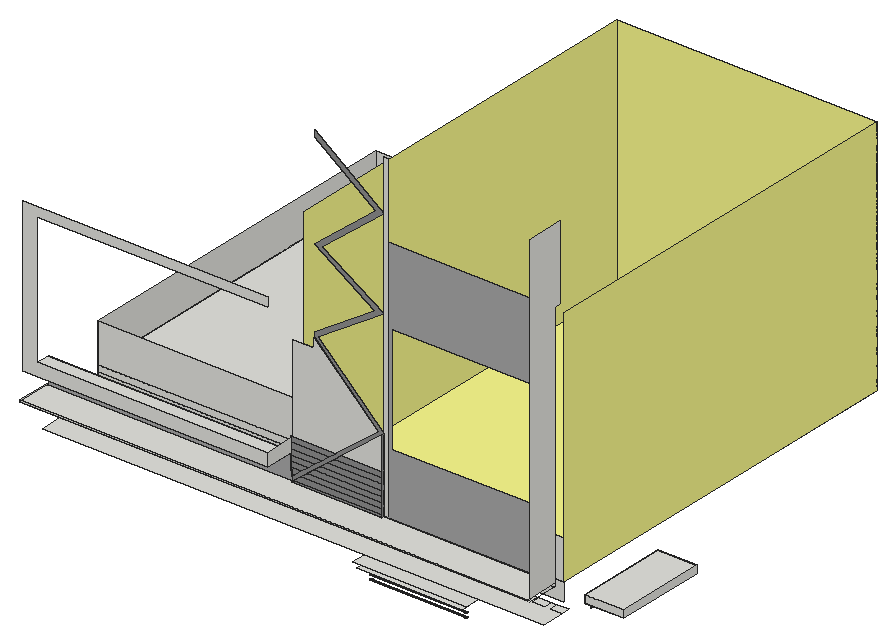
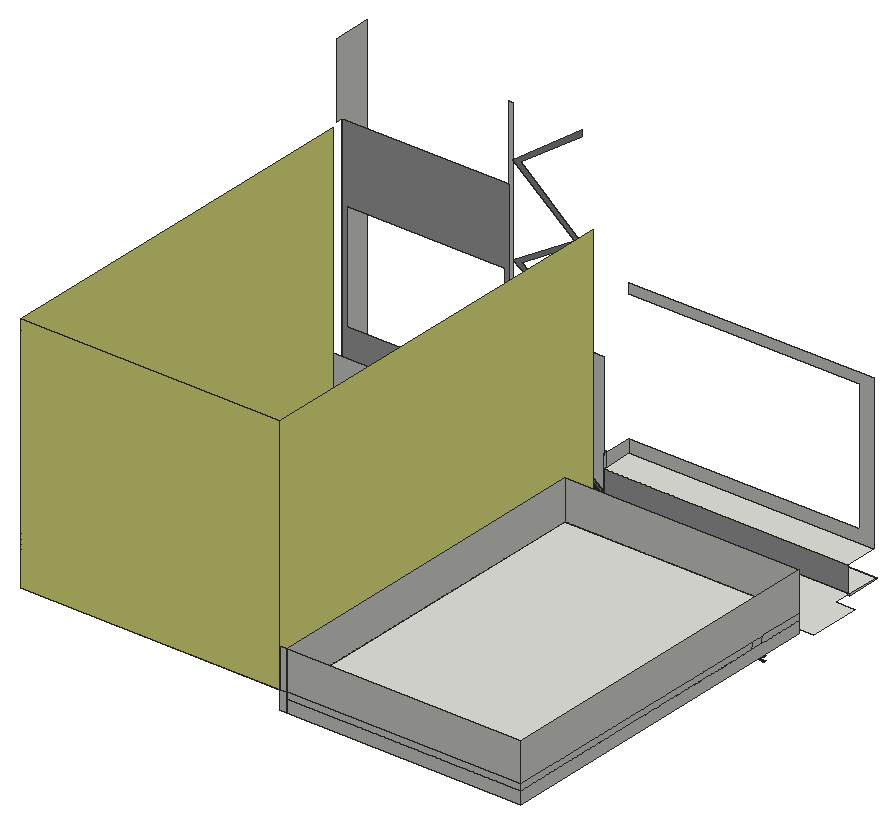
# SketchUp Ruby script. Lengths in inches.
U = 1.inch
M = Sketchup.active_model
def pt(a) = Geom::Point3d.new(a.map { |v| v * U })
def face(e, loops, mat)
  f = e.add_face(loops[0].map { |a| pt(a) })
  loops[1..].each { |l| e.add_face(l.map { |a| pt(a) }).erase! }
  f.material = f.back_material = mat if mat
  f
end
# faces: each face lists its corners as indices into pts; further lists are holes
def faces(e, pts, list, mat = nil) = list.each { |f| face(e, (f[0].is_a?(Array) ? f : [f]).map { |l| l.map { |i| pts[i] } }, mat) }
# xy, xz, yz: faces in a plane at the given z, y or x. An outline is a flat list of corners, or four numbers for a rectangle; further outlines are holes
def ring(l) = l.size == 4 ? [[l[0], l[1]], [l[2], l[1]], [l[2], l[3]], [l[0], l[3]]] : l.each_slice(2).to_a
def flat(e, list, mat, &to3) = list.each { |f| face(e, (f[0].is_a?(Array) ? f : [f]).map { |l| ring(l).map { |u, v| to3.(u, v) } }, mat) }
def xy(e, z, list, mat = nil) = flat(e, list, mat) { |x, y| [x, y, z] }
def xz(e, y, list, mat = nil) = flat(e, list, mat) { |x, z| [x, y, z] }
def yz(e, x, list, mat = nil) = flat(e, list, mat) { |y, z| [x, y, z] }
def lines(e, pts, list) = list.each { |a, b| e.add_line(pt(pts[a]), pt(pts[b])) }
# prism: a flat outline (further loops are holes) pulled along v
def prism(e, loops, v, mat = nil)
  f = face(e, loops, mat); d = Geom::Vector3d.new(v.map { |x| x * U })
  f.pushpull(f.normal.samedirection?(d) ? d.length : -d.length)
end
def box(e, o, s, mat = nil) = prism(e, [[o, [o[0] + s[0], o[1], o[2]], [o[0] + s[0], o[1] + s[1], o[2]], [o[0], o[1] + s[1], o[2]]]], [0, 0, s[2]], mat)
def at(x, y, z, deg = 0) = Geom::Transformation.translation(pt([x, y, z])) * Geom::Transformation.rotation(ORIGIN, Z_AXIS, deg.degrees)
def axes(o, x, y, z) = Geom::Transformation.new([*x, 0, *y, 0, *z, 0, *pt(o).to_a, 1])
def part(name) = M.definitions.add(name)
# library, detail: a bought-in or finely detailed component or shape, given as its bounding box
def library(name, o, s) = part(name).tap { |d| box(d.entities, o, s) }
def detail(e, o, s) = box(e.add_group.entities, o, s)
def put(e, d, t, mat = nil) = e.add_instance(d, t).tap { |i| i.material = mat if mat }
def group(e, t, mat = nil) = e.add_group.tap { |g| g.transformation = t; g.material = mat if mat }.entities
root = M.entities
M.materials.add("[0032_Moccasin]").color = [249, 249, 141]
M.materials.add("[0132_LightGray]").color = [169, 169, 169]
M.materials.add("[Color M04]").color = [142, 142, 142]
M.materials.add("[Wood Bamboo]").color = [195, 96, 5]
M.materials.add("[Wood Cherry Original]").color = [152, 68, 0]
M.materials.add("[Wood Cherry Original]1").color = [152, 86, 42]
xy(root,126,[[149.49,84.25,191.49,85.25]],"[Wood Cherry Original]")
xy(root,136.59,[[316.01,39.5625,334.01,43],[334.01,39.5625,340.01,40.5625],[340.01,39.5625,381.26,43],[381.26,39.5625,387.26,40.5625],[387.26,39.5625,405.26,43]],"[Wood Bamboo]")
xy(root,137.01,[[103.25,82.25,107.25,84.25]])
xy(root,137.01,[[61.9375,82.25,103.25,84.25],[107.25,82.25,119.25,84.25]],"[Wood Cherry Original]")
xy(root,140.59,[[312.01,30.4375,409.26,39.5625],[312.01,39.5625,409.26,43],[312.01,43,409.26,50.6875]])
xy(root,141.01,[[57.9375,82.25,123.25,84.25]],"[Wood Cherry Original]1")
xy(root,144.4,[[308.2,30.4375,413.0625,44.6875]])
xy(root,155,[[495.875,70.375,496.875,140.375]])
xy(root,162,[[495.875,63.375,496.875,147.375],[[496.875,63.375,531.875,147.375],[513.08,87.9375,514.63,88.14,516.08,88.74,517.32,89.7,518.28,90.9375,518.875,92.39,519.08,93.9375,518.875,95.49,518.28,96.9375,517.32,98.18,516.08,99.14,514.63,99.73,513.08,99.9375,511.53,99.73,510.08,99.14,508.84,98.18,507.88,96.9375,507.29,95.49,507.08,93.9375,507.29,92.39,507.88,90.9375,508.84,89.7,510.08,88.74,511.53,88.14]],[513.08,87.9375,511.53,88.14,510.08,88.74,508.84,89.7,507.88,90.9375,507.29,92.39,507.08,93.9375,507.29,95.49,507.88,96.9375,508.84,98.18,510.08,99.14,511.53,99.73,513.08,99.9375,514.63,99.73,516.08,99.14,517.32,98.18,518.28,96.9375,518.875,95.49,519.08,93.9375,518.875,92.39,518.28,90.9375,517.32,89.7,516.08,88.74,514.63,88.14]])
xy(root,165,[[33.875,15.6875,33.875,36.73,15.875,36.73,15.875,84.25,213.63,84.25,213.63,36.625,225.4375,36.625,225.4375,49.4375,230.75,49.4375,230.75,36.625,241.25,36.625,241.25,44.6875,468.26,44.6875,468.26,36.625,480.0625,36.625,480.0625,44.6875,485.375,44.6875,485.375,36.625,495.875,36.625,495.875,15.6875],[213.63,36.625,225.4375,84.25],[230.75,36.625,241.25,84.25],[468.26,36.625,480.0625,44.6875],[485.375,36.625,495.875,44.6875],
  [225.4375,49.4375,230.75,84.25]])
xy(root,169,[[495.875,63.375,531.875,147.375]])
xy(root,176,[[24.875,90.25,241.25,411]])
xy(root,180.75,[[14.3125,14.25,14.3125,44.6875,15.875,44.6875,15.875,15.6875,482.9375,15.6875,482.9375,14.25]])
xy(root,182,[[14.3125,14.25,482.9375,14.25,482.9375,44.6875,325.49,44.6875,325.49,42.75,241.89,42.75,241.89,44.6875,14.3125,44.6875],[241.89,42.75,325.49,44.6875],[241.89,44.6875,325.49,46.6875],[241.89,46.6875,241.89,52.125,247.25,52.125,247.25,50.6875,325.49,50.6875,325.49,46.6875],[247.25,50.6875,325.49,52.125],
  [24.875,90.25,241.25,411]])
xy(root,182,[[325.49,50.6875,486.875,50.6875,486.875,411,247.25,411,247.25,52.125,325.49,52.125]],"[0032_Moccasin]")
xy(root,205.89,[[15.875,15.6875,241.25,44.6875]])
xz(root,14.25,[[14.3125,180.75,482.9375,182]])
xz(root,15.6875,[[15.875,205.89,241.25,205.89,241.25,218,28.03,218,28.03,338,241.25,338,241.25,347,15.875,347]])
xz(root,42.75,[[241.89,182,325.49,182,325.49,183.79,244.08,183.79],[244.08,183.79,325.49,183.79,325.49,188.92,250.33,188.92],[241.76,186.7,244.49,188.92,241.7,188.92],[241.7,188.92,244.49,188.92,250.79,194.04,241.57,194.04],[250.33,188.92,325.49,188.92,325.49,194.04,256.59,194.04],
  [241.57,194.04,250.79,194.04,257.1,199.17,241.43,199.17],[256.59,194.04,325.49,194.04,325.49,199.17,262.85,199.17],[241.43,199.17,257.1,199.17,263.4,204.29,241.29,204.29],[262.85,199.17,325.49,199.17,325.49,204.29,269.11,204.29],[241.29,204.29,263.4,204.29,269.7,209.42,241.25,209.42,241.25,205.89],
  [269.11,204.29,325.49,204.29,325.49,209.42,275.37,209.42],[241.25,209.42,269.7,209.42,276,214.54,241.25,214.54],[275.37,209.42,325.49,209.42,325.49,214.54,281.625,214.54],[241.25,214.54,276,214.54,282.3,219.67,241.25,219.67],[281.625,214.54,325.49,214.54,325.49,219.67,287.88,219.67]],"[Color M04]")
xz(root,44.4375,[[241.76,186.7,241.25,205.89,241.25,298.5,261.37,298.5,261.37,306.96,319.9,250.25]])
xz(root,44.6875,[[325.49,179.25,329.48,182],[329.48,179.25,482.9375,182],[14.3125,180.75,15.875,182],[241.89,182,325.49,250.46,325.49,182],[325.49,182,329.48,479],
  [241.76,186.7,241.25,205.89,241.25,298.5,261.37,298.5,261.37,306.96,319.9,250.25]])
xz(root,44.6875,[[15.875,182,241.89,182,241.76,186.7,241.25,205.89,15.875,205.89],[[329.48,182,482.9375,410],[333.13,239.94,333.13,337.75,332.44,337.75,332.44,339.8125,478.87,339.8125,478.87,337.75,478.31,337.75,478.31,239.94]]],"[0132_LightGray]")
xz(root,44.6875,[[241.89,182,325.49,250.46,264.35,308.92,325.49,349.15,268.3,384.6,325.49,431.84,261.37,479,261.37,473.32,318.21,432.15,261.37,384.6,317.38,349.1,261.37,311.77,261.37,306.96,319.9,250.25,241.76,186.7]],"[Color M04]")
xz(root,46.6875,[[241.89,182,325.49,250.46,325.49,182]])
xz(root,50.6875,[[247.25,165,377.96,182],[377.96,165,403.71,182],[403.71,165,486.875,182],[247.25,182,486.875,218]])
xz(root,52.125,[[241.89,182,325.49,250.46,325.49,182]])
xz(root,63.375,[[495.875,162,531.875,169]])
xz(root,90.25,[[24.875,165,241.25,176],[24.875,176,241.25,182],[24.875,182,241.25,218]])
xz(root,147.375,[[495.875,162,531.875,169]])
xz(root,411,[[24.875,165,241.25,176],[241.25,165,247.25,182],[24.875,176,241.25,182],[24.875,182,241.25,218],[241.25,182,247.25,218]])
xz(root,411,[[247.25,182,486.875,404]],"[0032_Moccasin]")
yz(root,14.3125,[[14.25,180.75,44.6875,182]])
yz(root,24.875,[[90.25,165,411,176],[90.25,176,132.85,182],[132.85,176,144.6,182],[144.6,176,411,182],[90.25,182,411,218]])
yz(root,241.25,[[90.25,165,411,176],[90.25,176,411,182],[90.25,182,411,218],[15.6875,205.89,42.75,218],[42.75,205.89,44.4375,218],
  [44.4375,205.89,44.6875,218]])
yz(root,247.25,[[50.6875,182,411,404]],"[0032_Moccasin]")
yz(root,325.49,[[44.6875,182,46.6875,250.46],[46.6875,182,52.125,250.46]])
yz(root,325.49,[[42.75,182,44.6875,250.46]],"[Color M04]")
yz(root,482.9375,[[14.25,180.75,15.6875,182],[15.6875,182,15.6875,479,50.6875,479,50.6875,410,44.6875,410,44.6875,182]])
yz(root,486.875,[[50.6875,182,411,404]],"[0032_Moccasin]")
yz(root,495.875,[[63.375,162,147.375,169]])
yz(root,531.875,[[63.375,162,147.375,169]])
p = [[119.25,83,126.03],[119.25,82.9,126.11],[61.9375,82.9,126.11],[61.9375,83,126.03],[119.25,83.12,125.98],[61.9375,83.12,125.98],
  [119.25,83.25,125.96],[61.9375,83.25,125.96],[119.25,83.38,125.98],[61.9375,83.38,125.98],[119.25,83.5,126.03],[61.9375,83.5,126.03],
  [119.25,83.6,126.11],[61.9375,83.6,126.11],[119.25,82.82,126.21],[61.9375,82.82,126.21],[119.25,83.68,126.21],[61.9375,83.68,126.21],
  [119.25,82.77,126.34],[61.9375,82.77,126.34],[119.25,83.73,126.34],[61.9375,83.73,126.34],[119.25,82.75,126.46],[61.9375,82.75,126.46],
  [119.25,83.75,126.46],[61.9375,83.75,126.46],[119.25,82.77,126.59],[61.9375,82.77,126.59],[119.25,83.73,126.59],[61.9375,83.73,126.59],
  [119.25,82.82,126.71],[61.9375,82.82,126.71],[119.25,83.68,126.71],[61.9375,83.68,126.71],[119.25,82.9,126.82],[61.9375,82.9,126.82],
  [119.25,83.6,126.82],[61.9375,83.6,126.82],[119.25,83,126.9],[61.9375,83,126.9],[119.25,83.5,126.9],[61.9375,83.5,126.9],
  [119.25,83.12,126.95],[61.9375,83.12,126.95],[119.25,83.25,126.96],[61.9375,83.25,126.96],[119.25,83.38,126.95],[61.9375,83.38,126.95],
  [316.01,41.03,127.78],[316.01,41.15,127.73],[405.26,41.15,127.73],[405.26,41.03,127.78],[316.01,41.28,127.71],[405.26,41.28,127.71],
  [316.01,41.41,127.73],[405.26,41.41,127.73],[316.01,41.53,127.78],[405.26,41.53,127.78],[316.01,40.93,127.86],[405.26,40.93,127.86],
  [316.01,41.63,127.86],[405.26,41.63,127.86],[316.01,40.85,127.96],[405.26,40.85,127.96],[316.01,41.71,127.96],[405.26,41.71,127.96],
  [316.01,40.8,128.08],[405.26,40.8,128.08],[316.01,41.76,128.08],[405.26,41.76,128.08],[316.01,40.78,128.21],[405.26,40.78,128.21],
  [316.01,41.78,128.21],[405.26,41.78,128.21],[316.01,40.8,128.34],[405.26,40.8,128.34],[316.01,41.76,128.34],[405.26,41.76,128.34],
  [316.01,40.85,128.46],[405.26,40.85,128.46],[316.01,41.71,128.46],[405.26,41.71,128.46],[316.01,40.93,128.57],[405.26,40.93,128.57],
  [316.01,41.63,128.57],[405.26,41.63,128.57],[316.01,41.03,128.65],[405.26,41.03,128.65],[316.01,41.15,128.7],[405.26,41.15,128.7],
  [316.01,41.53,128.65],[316.01,41.41,128.7],[405.26,41.41,128.7],[405.26,41.53,128.65],[316.01,41.28,128.71],[405.26,41.28,128.71],
  [119.25,83,130.03],[119.25,82.9,130.11],[61.9375,82.9,130.11],[61.9375,83,130.03],[119.25,83.12,129.98],[61.9375,83.12,129.98],
  [119.25,83.25,129.96],[61.9375,83.25,129.96],[119.25,83.38,129.98],[61.9375,83.38,129.98],[119.25,83.5,130.03],[61.9375,83.5,130.03],
  [119.25,83.6,130.11],[61.9375,83.6,130.11],[119.25,82.82,130.21],[61.9375,82.82,130.21],[119.25,83.68,130.21],[61.9375,83.68,130.21],
  [119.25,82.77,130.34],[61.9375,82.77,130.34],[119.25,83.73,130.34],[61.9375,83.73,130.34],[119.25,82.75,130.46],[61.9375,82.75,130.46],
  [119.25,83.75,130.46],[61.9375,83.75,130.46],[119.25,82.77,130.59],[61.9375,82.77,130.59],[119.25,83.73,130.59],[61.9375,83.73,130.59],
  [119.25,82.82,130.71],[61.9375,82.82,130.71],[119.25,83.68,130.71],[61.9375,83.68,130.71],[119.25,82.9,130.82],[61.9375,82.9,130.82],
  [119.25,83.6,130.82],[61.9375,83.6,130.82],[119.25,83,130.9],[61.9375,83,130.9],[119.25,83.5,130.9],[61.9375,83.5,130.9],
  [119.25,83.12,130.95],[61.9375,83.12,130.95],[119.25,83.25,130.96],[61.9375,83.25,130.96],[119.25,83.38,130.95],[61.9375,83.38,130.95],
  [316.01,41.03,131.78],[316.01,41.15,131.73],[405.26,41.15,131.73],[405.26,41.03,131.78],[316.01,41.28,131.71],[405.26,41.28,131.71],
  [316.01,41.41,131.73],[405.26,41.41,131.73],[316.01,41.53,131.78],[405.26,41.53,131.78],[316.01,40.93,131.86],[405.26,40.93,131.86],
  [316.01,41.63,131.86],[405.26,41.63,131.86],[316.01,40.85,131.96],[405.26,40.85,131.96],[316.01,41.71,131.96],[405.26,41.71,131.96],
  [316.01,40.8,132.08],[405.26,40.8,132.08],[316.01,41.76,132.08],[405.26,41.76,132.08],[316.01,40.78,132.21],[405.26,40.78,132.21],
  [316.01,41.78,132.21],[405.26,41.78,132.21],[316.01,40.8,132.34],[405.26,40.8,132.34],[316.01,41.76,132.34],[405.26,41.76,132.34],
  [316.01,40.85,132.46],[405.26,40.85,132.46],[316.01,41.71,132.46],[405.26,41.71,132.46],[316.01,40.93,132.57],[405.26,40.93,132.57],
  [316.01,41.63,132.57],[405.26,41.63,132.57],[316.01,41.03,132.65],[405.26,41.03,132.65],[316.01,41.15,132.7],[405.26,41.15,132.7],
  [316.01,41.53,132.65],[316.01,41.41,132.7],[405.26,41.41,132.7],[405.26,41.53,132.65],[316.01,41.28,132.71],[405.26,41.28,132.71],
  [119.25,83,134.03],[119.25,82.9,134.11],[61.9375,82.9,134.11],[61.9375,83,134.03],[119.25,83.12,133.98],[61.9375,83.12,133.98],
  [119.25,83.25,133.96],[61.9375,83.25,133.96],[119.25,83.38,133.98],[61.9375,83.38,133.98],[119.25,83.5,134.03],[61.9375,83.5,134.03],
  [119.25,83.6,134.11],[61.9375,83.6,134.11],[119.25,82.82,134.21],[61.9375,82.82,134.21],[119.25,83.68,134.21],[61.9375,83.68,134.21],
  [119.25,82.77,134.34],[61.9375,82.77,134.34],[119.25,83.73,134.34],[61.9375,83.73,134.34],[119.25,82.75,134.46],[61.9375,82.75,134.46],
  [119.25,83.75,134.46],[61.9375,83.75,134.46],[119.25,82.77,134.59],[61.9375,82.77,134.59],[119.25,83.73,134.59],[61.9375,83.73,134.59],
  [119.25,82.82,134.71],[61.9375,82.82,134.71],[119.25,83.68,134.71],[61.9375,83.68,134.71],[119.25,82.9,134.82],[61.9375,82.9,134.82],
  [119.25,83.6,134.82],[61.9375,83.6,134.82],[119.25,83,134.9],[61.9375,83,134.9],[119.25,83.5,134.9],[61.9375,83.5,134.9],
  [119.25,83.12,134.95],[61.9375,83.12,134.95],[119.25,83.25,134.96],[61.9375,83.25,134.96],[119.25,83.38,134.95],[61.9375,83.38,134.95],
  [325.49,44.6875,250.46],[241.89,44.6875,182],[241.89,42.75,182],[244.08,42.75,183.79],[250.33,42.75,188.92],[256.59,42.75,194.04],
  [262.85,42.75,199.17],[269.11,42.75,204.29],[275.37,42.75,209.42],[281.625,42.75,214.54],[287.88,42.75,219.67],[294.14,42.75,224.79],
  [300.4,42.75,229.92],[306.66,42.75,235.04],[312.92,42.75,240.17],[319.17,42.75,245.29],[325.43,42.75,250.42],[325.49,42.75,250.46],
  [325.49,46.6875,250.46],[241.89,46.6875,182],[241.89,52.125,182],[325.49,52.125,250.46],[241.29,42.75,204.29],[241.25,42.75,205.89],
  [241.25,44.4375,205.89],[241.76,44.4375,186.7],[241.76,42.75,186.7],[241.7,42.75,188.92],[241.57,42.75,194.04],[241.43,42.75,199.17],
  [319.9,42.75,250.25],[313.81,42.75,245.29],[307.51,42.75,240.17],[301.2,42.75,235.04],[294.9,42.75,229.92],[288.6,42.75,224.79],
  [282.3,42.75,219.67],[276,42.75,214.54],[269.7,42.75,209.42],[263.4,42.75,204.29],[257.1,42.75,199.17],[250.79,42.75,194.04],
  [244.49,42.75,188.92],[319.9,44.4375,250.25],[241.25,44.6875,205.89],[241.76,44.6875,186.7],[319.9,44.6875,250.25],[482.9375,44.6875,179.25],
  [482.9375,15.6875,179.25],[265.5625,42.75,178.67],[325.49,42.75,178.67],[265.5625,42.75,173.54],[325.49,42.75,173.54],[265.5625,42.75,168.42],
  [325.49,42.75,168.42],[241.25,42.75,204.29]]
faces(root,p,[[0,1,2,3],[4,0,3,5],[6,4,5,7],[8,6,7,9],[10,8,9,11],[12,10,11,13],[1,14,15,2],[16,12,13,17],
  [14,18,19,15],[20,16,17,21],[18,22,23,19],[24,20,21,25],[22,26,27,23],[28,24,25,29],[26,30,31,27],[32,28,29,33],
  [30,34,35,31],[36,32,33,37],[34,38,39,35],[40,36,37,41],[38,42,43,39],[42,44,45,43],[44,46,47,45],[46,40,41,47],
  [48,49,50,51],[49,52,53,50],[52,54,55,53],[54,56,57,55],[58,48,51,59],[56,60,61,57],[62,58,59,63],[60,64,65,61],
  [66,62,63,67],[64,68,69,65],[70,66,67,71],[68,72,73,69],[74,70,71,75],[72,76,77,73],[78,74,75,79],[76,80,81,77],
  [82,78,79,83],[80,84,85,81],[86,82,83,87],[88,86,87,89],[90,91,92,93],[84,90,93,85],[94,88,89,95],[91,94,95,92],
  [96,97,98,99],[100,96,99,101],[102,100,101,103],[104,102,103,105],[106,104,105,107],[108,106,107,109],[97,110,111,98],[112,108,109,113],
  [110,114,115,111],[116,112,113,117],[114,118,119,115],[120,116,117,121],[118,122,123,119],[124,120,121,125],[122,126,127,123],[128,124,125,129],
  [126,130,131,127],[132,128,129,133],[130,134,135,131],[136,132,133,137],[134,138,139,135],[138,140,141,139],[140,142,143,141],[142,136,137,143],
  [144,145,146,147],[145,148,149,146],[148,150,151,149],[150,152,153,151],[154,144,147,155],[152,156,157,153],[158,154,155,159],[156,160,161,157],
  [162,158,159,163],[160,164,165,161],[166,162,163,167],[164,168,169,165],[170,166,167,171],[168,172,173,169],[174,170,171,175],[172,176,177,173],
  [178,174,175,179],[176,180,181,177],[182,178,179,183],[184,182,183,185],[186,187,188,189],[180,186,189,181],[190,184,185,191],[187,190,191,188],
  [192,193,194,195],[196,192,195,197],[198,196,197,199],[200,198,199,201],[202,200,201,203],[204,202,203,205],[193,206,207,194],[208,204,205,209],
  [206,210,211,207],[212,208,209,213],[210,214,215,211],[216,212,213,217],[214,218,219,215],[220,216,217,221],[218,222,223,219],[224,220,221,225],
  [222,226,227,223],[228,224,225,229],[226,230,231,227],[232,228,229,233],[230,234,235,231],[234,236,237,235],[236,238,239,237],[238,232,233,239]],"[0132_LightGray]")
faces(root,p,[[240,241,242,243,244,245,246,247,248,249,250,251,252,253,254,255,256,257],[270,271,272,273,274,275,276,277,278,279,280,281,282,266,265,283]],"[Color M04]")
faces(root,p,[[241,240,258,259],[260,259,258,261],[262,263,264,265,266,267,268,269],[284,285,265,264],[285,286,283,265]])
lines(root,p,[[287,288],[289,290],[291,292],[293,294],[262,295]])
